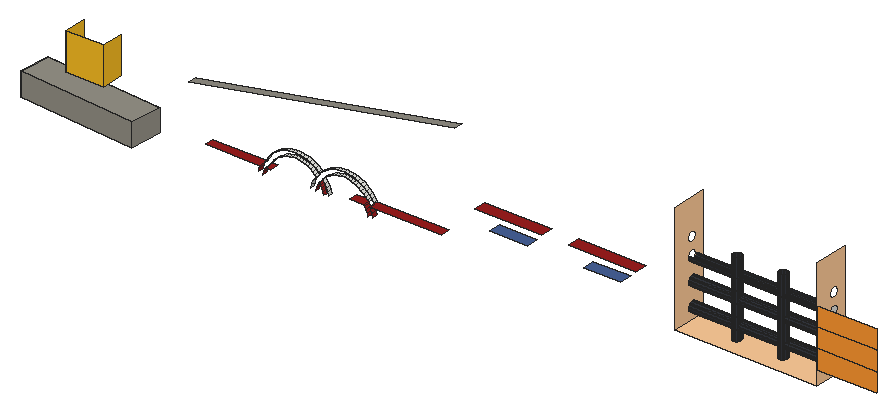
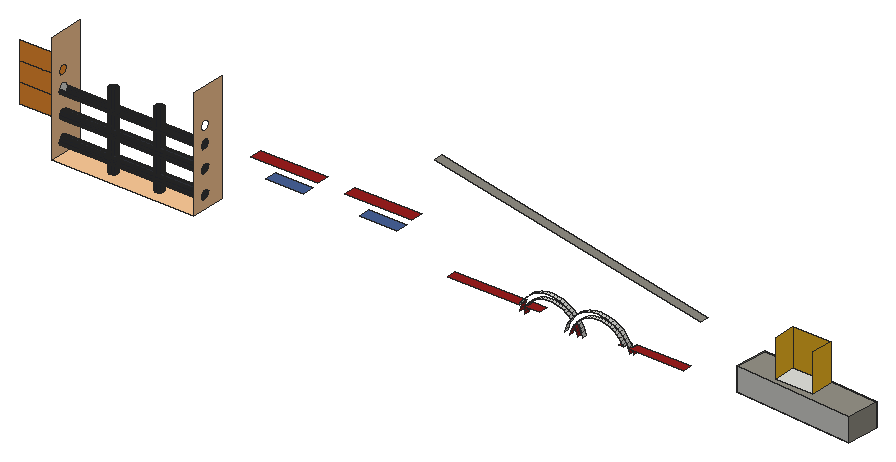
# SketchUp Ruby script. Lengths in inches.
U = 1.inch
M = Sketchup.active_model
def pt(a) = Geom::Point3d.new(a.map { |v| v * U })
def face(e, loops, mat)
  f = e.add_face(loops[0].map { |a| pt(a) })
  loops[1..].each { |l| e.add_face(l.map { |a| pt(a) }).erase! }
  f.material = f.back_material = mat if mat
  f
end
# faces: each face lists its corners as indices into pts; further lists are holes
def faces(e, pts, list, mat = nil) = list.each { |f| face(e, (f[0].is_a?(Array) ? f : [f]).map { |l| l.map { |i| pts[i] } }, mat) }
# xy, xz, yz: faces in a plane at the given z, y or x. An outline is a flat list of corners, or four numbers for a rectangle; further outlines are holes
def ring(l) = l.size == 4 ? [[l[0], l[1]], [l[2], l[1]], [l[2], l[3]], [l[0], l[3]]] : l.each_slice(2).to_a
def flat(e, list, mat, &to3) = list.each { |f| face(e, (f[0].is_a?(Array) ? f : [f]).map { |l| ring(l).map { |u, v| to3.(u, v) } }, mat) }
def xy(e, z, list, mat = nil) = flat(e, list, mat) { |x, y| [x, y, z] }
def xz(e, y, list, mat = nil) = flat(e, list, mat) { |x, z| [x, y, z] }
def yz(e, x, list, mat = nil) = flat(e, list, mat) { |y, z| [x, y, z] }
def lines(e, pts, list) = list.each { |a, b| e.add_line(pt(pts[a]), pt(pts[b])) }
# prism: a flat outline (further loops are holes) pulled along v
def prism(e, loops, v, mat = nil)
  f = face(e, loops, mat); d = Geom::Vector3d.new(v.map { |x| x * U })
  f.pushpull(f.normal.samedirection?(d) ? d.length : -d.length)
end
def box(e, o, s, mat = nil) = prism(e, [[o, [o[0] + s[0], o[1], o[2]], [o[0] + s[0], o[1] + s[1], o[2]], [o[0], o[1] + s[1], o[2]]]], [0, 0, s[2]], mat)
def at(x, y, z, deg = 0) = Geom::Transformation.translation(pt([x, y, z])) * Geom::Transformation.rotation(ORIGIN, Z_AXIS, deg.degrees)
def axes(o, x, y, z) = Geom::Transformation.new([*x, 0, *y, 0, *z, 0, *pt(o).to_a, 1])
def part(name) = M.definitions.add(name)
# library, detail: a bought-in or finely detailed component or shape, given as its bounding box
def library(name, o, s) = part(name).tap { |d| box(d.entities, o, s) }
def detail(e, o, s) = box(e.add_group.entities, o, s)
def put(e, d, t, mat = nil) = e.add_instance(d, t).tap { |i| i.material = mat if mat }
def group(e, t, mat = nil) = e.add_group.tap { |g| g.transformation = t; g.material = mat if mat }.entities
root = M.entities
M.materials.add("[0045_Goldenrod]").color = [249, 189, 36]
M.materials.add("[Color A04]").color = [155, 30, 30]
M.materials.add("[Color C02]").color = [255, 204, 153]
M.materials.add("[Color C04]").color = [255, 153, 50]
M.materials.add("[Formica Blue]").color = [71, 97, 152]
M.materials.add("[Formica Graystone]").color = [149, 146, 135]
M.materials.add("[Formica Laminate Dark]").color = [50, 53, 60]
xy(root,271.875,[[[383.64,94.74,470.23,116.19],[411.92,104.06,411.25,104.14,410.64,104.4,410.11,104.81,409.7,105.34,409.44,105.95,409.36,106.62,409.44,107.28,409.7,107.9,410.11,108.43,410.64,108.84,411.25,109.09,411.92,109.18,412.58,109.09,413.2,108.84,413.73,108.43,414.14,107.9,414.39,107.28,414.48,106.62,414.39,105.95,414.14,105.34,413.73,104.81,413.2,104.4,412.58,104.14],[440.11,104.06,439.44,104.14,438.82,104.4,438.29,104.81,437.89,105.34,437.63,105.95,437.54,106.62,437.63,107.28,437.89,107.9,438.29,108.43,438.82,108.84,439.44,109.09,440.11,109.18,440.77,109.09,441.39,108.84,441.92,108.43,442.32,107.9,442.58,107.28,442.67,106.62,442.58,105.95,442.32,105.34,441.92,104.81,441.39,104.4,440.77,104.14]]],"[Color C02]")
xy(root,272.99,[[72.23,70.04,0,75.36,1.43,94.74,73.65,89.43]])
xy(root,276.95,[[101.95,89.24,135.19,94.74],[138.52,89.24,141.51,94.74]],"[Color A04]")
xy(root,277.9375,[[189.67,89.24,198.57,94.74],[202,89.24,245.58,94.74]],"[Color A04]")
xy(root,287.03,[[72.23,70.04,73.65,89.43,1.43,94.74,0,75.36]],"[Formica Graystone]")
xy(root,291.97,[[276.8,87.3,299.68,94.74],[333.8,87.3,356.68,94.74]],"[Formica Blue]")
xy(root,292.05,[[23.1,81.43,45.78,94.74]])
xy(root,300.97,[[267.8,87.3,308.68,94.74],[324.8,87.3,365.68,94.74]],"[Color A04]")
xz(root,81.43,[[23.1,292.05,45.78,314.74]],"[0045_Goldenrod]")
xz(root,94.74,[[470.23,280.78,506.36,292.4],[470.23,292.4,506.36,304.03],[470.23,304.03,506.36,315.65]],"[Color C04]")
yz(root,23.1,[[81.43,292.05,94.74,314.74]],"[0045_Goldenrod]")
yz(root,45.78,[[81.43,292.05,94.74,314.74]],"[0045_Goldenrod]")
yz(root,383.64,[[[94.74,271.875,116.19,338.91],[107.5,314.66,106.75,314.76,106.06,315.05,105.46,315.51,105.01,316.1,104.72,316.79,104.62,317.54,104.72,318.28,105.01,318.98,105.46,319.57,106.06,320.03,106.75,320.32,107.5,320.41,108.24,320.32,108.93,320.03,109.53,319.57,109.99,318.98,110.27,318.28,110.37,317.54,110.27,316.79,109.99,316.1,109.53,315.51,108.93,315.05,108.24,314.76],[107.5,304.48,106.75,304.57,106.06,304.86,105.46,305.32,105.01,305.91,104.72,306.61,104.62,307.35,104.72,308.09,105.01,308.79,105.46,309.38,106.06,309.84,106.75,310.13,107.5,310.23,108.24,310.13,108.93,309.84,109.53,309.38,109.99,308.79,110.27,308.09,110.37,307.35,110.27,306.61,109.99,305.91,109.53,305.32,108.93,304.86,108.24,304.57],[107.5,290.91,106.75,291.01,106.06,291.3,105.46,291.76,105.01,292.35,104.72,293.04,104.62,293.79,104.72,294.53,105.01,295.23,105.46,295.82,106.06,296.28,106.75,296.57,107.5,296.66,108.24,296.57,108.93,296.28,109.53,295.82,109.99,295.23,110.27,294.53,110.37,293.79,110.27,293.04,109.99,292.35,109.53,291.76,108.93,291.3,108.24,291.01],[107.5,276.73,106.75,276.82,106.06,277.11,105.46,277.57,105.01,278.16,104.72,278.86,104.62,279.6,104.72,280.34,105.01,281.04,105.46,281.63,106.06,282.09,106.75,282.38,107.5,282.48,108.24,282.38,108.93,282.09,109.53,281.63,109.99,281.04,110.27,280.34,110.37,279.6,110.27,278.86,109.99,278.16,109.53,277.57,108.93,277.11,108.24,276.82]]],"[Color C02]")
yz(root,470.23,[[107.5,276.73,108.24,276.82,108.93,277.11,109.53,277.57,109.99,278.16,110.27,278.86,110.37,279.6,110.27,280.34,109.99,281.04,109.53,281.63,108.93,282.09,108.24,282.38,107.5,282.48,106.75,282.38,106.06,282.09,105.46,281.63,105.01,281.04,104.72,280.34,104.62,279.6,104.72,278.86,105.01,278.16,105.46,277.57,106.06,277.11,106.75,276.82],[107.5,290.91,108.24,291.01,108.93,291.3,109.53,291.76,109.99,292.35,110.27,293.04,110.37,293.79,110.27,294.53,109.99,295.23,109.53,295.82,108.93,296.28,108.24,296.57,107.5,296.66,106.75,296.57,106.06,296.28,105.46,295.82,105.01,295.23,104.72,294.53,104.62,293.79,104.72,293.04,105.01,292.35,105.46,291.76,106.06,291.3,106.75,291.01],[107.5,304.48,108.24,304.57,108.93,304.86,109.53,305.32,109.99,305.91,110.27,306.61,110.37,307.35,110.27,308.09,109.99,308.79,109.53,309.38,108.93,309.84,108.24,310.13,107.5,310.23,106.75,310.13,106.06,309.84,105.46,309.38,105.01,308.79,104.72,308.09,104.62,307.35,104.72,306.61,105.01,305.91,105.46,305.32,106.06,304.86,106.75,304.57]])
yz(root,470.23,[[[94.74,271.875,116.19,338.91],[107.5,276.73,108.24,276.82,108.93,277.11,109.53,277.57,109.99,278.16,110.27,278.86,110.37,279.6,110.27,280.34,109.99,281.04,109.53,281.63,108.93,282.09,108.24,282.38,107.5,282.48,106.75,282.38,106.06,282.09,105.46,281.63,105.01,281.04,104.72,280.34,104.62,279.6,104.72,278.86,105.01,278.16,105.46,277.57,106.06,277.11,106.75,276.82],[107.5,290.91,108.24,291.01,108.93,291.3,109.53,291.76,109.99,292.35,110.27,293.04,110.37,293.79,110.27,294.53,109.99,295.23,109.53,295.82,108.93,296.28,108.24,296.57,107.5,296.66,106.75,296.57,106.06,296.28,105.46,295.82,105.01,295.23,104.72,294.53,104.62,293.79,104.72,293.04,105.01,292.35,105.46,291.76,106.06,291.3,106.75,291.01],[107.5,304.48,108.24,304.57,108.93,304.86,109.53,305.32,109.99,305.91,110.27,306.61,110.37,307.35,110.27,308.09,109.99,308.79,109.53,309.38,108.93,309.84,108.24,310.13,107.5,310.23,106.75,310.13,106.06,309.84,105.46,309.38,105.01,308.79,104.72,308.09,104.62,307.35,104.72,306.61,105.01,305.91,105.46,305.32,106.06,304.86,106.75,304.57],[107.5,314.66,108.24,314.76,108.93,315.05,109.53,315.51,109.99,316.1,110.27,316.79,110.37,317.54,110.27,318.28,109.99,318.98,109.53,319.57,108.93,320.03,108.24,320.32,107.5,320.41,106.75,320.32,106.06,320.03,105.46,319.57,105.01,318.98,104.72,318.28,104.62,317.54,104.72,316.79,105.01,316.1,105.46,315.51,106.06,315.05,106.75,314.76]]],"[Color C02]")
p = [[410.64,104.4,271.875],[411.25,104.14,271.875],[411.25,104.14,317.54],[410.64,104.4,317.54],[411.92,104.06,271.875],[411.92,104.06,317.54],
  [412.58,104.14,271.875],[412.58,104.14,317.54],[413.2,104.4,271.875],[413.2,104.4,317.54],[438.82,104.4,271.875],[439.44,104.14,271.875],
  [439.44,104.14,318.0625],[438.82,104.4,318.0625],[440.11,104.06,271.875],[440.11,104.06,318.0625],[440.77,104.14,271.875],[440.77,104.14,318.0625],
  [441.39,104.4,271.875],[441.39,104.4,318.0625],[410.11,104.81,271.875],[410.35,104.62,317.54],[410.11,104.81,317.54],[413.73,104.81,271.875],
  [413.73,104.81,317.54],[413.49,104.62,317.54],[438.29,104.81,271.875],[438.29,104.81,318.0625],[441.92,104.81,271.875],[441.92,104.81,318.0625],
  [409.7,105.34,271.875],[409.7,105.34,317.54],[414.14,105.34,271.875],[414.14,105.34,317.54],[437.89,105.34,271.875],[437.89,105.34,318.0625],
  [442.32,105.34,271.875],[442.32,105.34,318.0625],[409.44,105.95,271.875],[409.44,105.95,317.54],[414.39,105.95,271.875],[414.39,105.95,317.54],
  [437.63,105.95,271.875],[437.63,105.95,318.0625],[442.58,105.95,271.875],[442.58,105.95,318.0625],[409.36,106.62,271.875],[409.36,106.62,317.54],
  [414.48,106.62,271.875],[414.48,106.62,317.54],[437.54,106.62,271.875],[437.54,106.62,318.0625],[442.67,106.62,271.875],[442.67,106.62,318.0625],
  [409.44,107.28,271.875],[409.44,107.28,317.54],[414.39,107.28,271.875],[414.39,107.28,317.54],[437.63,107.28,271.875],[437.63,107.28,318.0625],
  [442.58,107.28,271.875],[442.58,107.28,318.0625],[409.7,107.9,271.875],[409.7,107.9,317.54],[414.14,107.9,271.875],[414.14,107.9,317.54],
  [437.89,107.9,271.875],[437.89,107.9,318.0625],[442.32,107.9,271.875],[442.32,107.9,318.0625],[410.11,108.43,271.875],[410.11,108.43,317.54],
  [413.73,108.43,271.875],[413.73,108.43,317.54],[438.29,108.43,271.875],[438.29,108.43,318.0625],[441.92,108.43,271.875],[441.92,108.43,318.0625],
  [410.64,108.84,271.875],[410.64,108.84,317.54],[413.2,108.84,271.875],[413.2,108.84,317.54],[438.82,108.84,271.875],[438.82,108.84,318.0625],
  [441.39,108.84,271.875],[441.39,108.84,318.0625],[411.25,109.09,271.875],[411.25,109.09,317.54],[412.58,109.09,271.875],[412.58,109.09,317.54],
  [439.44,109.09,271.875],[439.44,109.09,318.0625],[440.77,109.09,271.875],[440.77,109.09,318.0625],[411.92,109.18,271.875],[411.92,109.18,317.54],
  [440.11,109.18,271.875],[440.11,109.18,318.0625],[200.89,92.37,272.03],[200.45,92.37,273.82],[200.45,89.24,273.82],[200.89,89.24,272.03],
  [170.95,94.74,273.82],[171.39,94.74,272.03],[171.39,92.37,272.03],[170.95,92.37,273.82],[203.32,92.37,274.6875],[203.84,92.37,272.59],
  [203.84,89.24,272.59],[203.32,89.24,274.6875],[174.34,94.74,272.59],[173.82,94.74,274.6875],[173.82,92.37,274.6875],[174.34,92.37,272.59],
  [136.92,92.37,272.73],[136.92,89.24,272.73],[137.43,89.24,274.51],[137.43,92.37,274.51],[166.42,94.74,272.73],[166.93,94.74,274.51],
  [166.93,92.37,274.51],[166.42,92.37,272.73],[72.23,70.04,287.03],[0,75.36,287.03],[0,75.36,272.99],[72.23,70.04,272.99],
  [73.65,89.43,272.99],[73.65,89.43,287.03],[1.43,94.74,287.03],[1.43,94.74,272.99],[134,92.37,273.42],[134.6,92.37,275.49],
  [134.6,89.24,275.49],[134,89.24,273.42],[164.1,94.74,275.49],[163.5,94.74,273.42],[163.5,92.37,273.42],[164.1,92.37,275.49],
  [199.82,92.37,275.55],[199.82,89.24,275.55],[170.32,94.74,275.55],[170.32,92.37,275.55],[138.13,89.24,276.21],[138.13,92.37,276.21],
  [167.63,94.74,276.21],[167.63,92.37,276.21],[202.59,92.37,276.72],[202.59,89.24,276.72],[173.09,94.74,276.72],[173.09,92.37,276.72],
  [135.19,92.37,276.95],[135.19,89.24,276.95],[164.91,94.74,277.49],[164.91,92.37,277.49],[199.02,92.37,277.21],[199.02,89.24,277.21],
  [169.52,94.74,277.21],[169.52,92.37,277.21],[138.52,89.24,276.95],[138.52,92.37,276.95],[168.5,94.74,277.84],[168.5,92.37,277.84],
  [202,92.37,277.9375],[202,89.24,277.9375],[172.15,94.74,278.66],[172.15,92.37,278.66],[470.23,107.5,276.73],[470.23,106.75,276.82],
  [383.64,106.75,276.82],[383.64,107.5,276.73],[470.23,108.24,276.82],[383.64,108.24,276.82],[470.23,106.06,277.11],[383.64,106.06,277.11],
  [470.23,108.93,277.11],[383.64,108.93,277.11],[135.41,94.74,277.49],[135.19,94.74,276.95],[135.41,92.37,277.49],[138.52,94.74,276.95],
  [139,94.74,277.84],[139,92.37,277.84],[470.23,105.46,277.57],[383.64,105.46,277.57],[470.23,109.53,277.57],[383.64,109.53,277.57],
  [198.57,92.37,277.9375],[198.57,89.24,277.9375],[168.83,94.74,278.32],[168.83,92.37,278.32],[136.43,94.74,279.39],[136.43,92.37,279.39],
  [165.93,94.74,279.39],[165.93,92.37,279.39],[470.23,105.01,278.16],[383.64,105.01,278.16],[470.23,109.99,278.16],[383.64,109.99,278.16],
  [140.04,94.74,279.37],[140.04,92.37,279.37],[198.04,94.74,278.78],[198.57,94.74,277.9375],[198.04,92.37,278.78],[202,94.74,277.9375],
  [201.65,94.74,278.66],[201.65,92.37,278.66],[470.23,104.72,278.86],[383.64,104.72,278.86],[470.23,110.27,278.86],[383.64,110.27,278.86],
  [171.01,94.74,280.5],[171.01,92.37,280.5],[200.51,94.74,280.5],[200.51,92.37,280.5],[196.91,94.74,280.24],[196.91,92.37,280.24],
  [470.23,104.62,279.6],[383.64,104.62,279.6],[470.23,110.37,279.6],[383.64,110.37,279.6],[137.64,94.74,281.18],[137.64,92.37,281.18],
  [141.23,94.74,280.78],[141.23,92.37,280.78],[166.88,94.74,280.79],[166.88,92.37,280.79],[470.23,104.72,280.34],[383.64,104.72,280.34],
  [470.23,110.27,280.34],[383.64,110.27,280.34],[195.64,94.74,281.57],[195.64,92.37,281.57],[470.23,105.01,281.04],[383.64,105.01,281.04],
  [470.23,109.99,281.04],[383.64,109.99,281.04],[170.76,94.74,280.8125],[170.76,92.37,280.8125],[199.19,94.74,282.2],[199.19,92.37,282.2],
  [142.56,94.74,282.05],[142.56,92.37,282.05],[166.14,94.74,281.57],[166.14,92.37,281.57],[172.06,94.74,282.05],[172.06,92.37,282.05],
  [470.23,105.46,281.63],[383.64,105.46,281.63],[470.23,109.53,281.63],[383.64,109.53,281.63],[139.04,94.74,282.83],[139.04,92.37,282.83],
  [164.73,94.74,282.76],[164.73,92.37,282.76],[194.23,94.74,282.76],[194.23,92.37,282.76],[470.23,106.06,282.09],[383.64,106.06,282.09],
  [470.23,108.93,282.09],[383.64,108.93,282.09],[144.01,94.74,283.18],[144.01,92.37,283.18],[173.51,94.74,283.18],[173.51,92.37,283.18],
  [470.23,106.75,282.38],[383.64,106.75,282.38],[470.23,108.24,282.38],[383.64,108.24,282.38],[197.69,94.74,283.76],[197.69,92.37,283.76],
  [470.23,107.5,282.48],[383.64,107.5,282.48],[140.59,94.74,284.32],[140.59,92.37,284.32],[163.2,94.74,283.8],[163.2,92.37,283.8],
  [192.7,94.74,283.8],[192.7,92.37,283.8],[168.82,94.74,283.1],[168.19,94.74,283.76],[168.19,92.37,283.76],[168.82,92.37,283.1],
  [170.09,94.74,284.32],[170.09,92.37,284.32],[145.58,94.74,284.16],[145.58,92.37,284.16],[175.08,94.74,284.16],[175.08,92.37,284.16],
  [161.57,94.74,284.67],[161.57,92.37,284.67],[166.54,94.74,285.15],[166.54,92.37,285.15],[191.07,94.74,284.67],[191.07,92.37,284.67],
  [196.04,94.74,285.15],[196.04,92.37,285.15],[147.24,94.74,284.96],[147.24,92.37,284.96],[176.74,94.74,284.96],[176.74,92.37,284.96],
  [142.3,94.74,285.65],[142.3,92.37,285.65],[171.8,94.74,285.65],[171.8,92.37,285.65],[159.87,94.74,285.36],[159.87,92.37,285.36],
  [189.37,94.74,285.36],[189.37,92.37,285.36],[148.98,94.74,285.59],[148.98,92.37,285.59],[178.48,94.74,285.59],[178.48,92.37,285.59],
  [164.75,94.74,286.36],[164.75,92.37,286.36],[194.25,94.74,286.36],[194.25,92.37,286.36],[158.09,94.74,285.88],[158.09,92.37,285.88],
  [187.59,94.74,285.88],[187.59,92.37,285.88],[144.13,94.74,286.79],[144.13,92.37,286.79],[150.77,94.74,286.03],[150.77,92.37,286.03],
  [173.63,94.74,286.79],[173.63,92.37,286.79],[180.27,94.74,286.03],[180.27,92.37,286.03],[156.28,94.74,286.2],[156.28,92.37,286.2],
  [185.78,94.74,286.2],[185.78,92.37,286.2],[152.6,94.74,286.28],[152.6,92.37,286.28],[182.1,94.74,286.28],[182.1,92.37,286.28],
  [154.4375,94.74,286.34],[154.4375,92.37,286.34],[183.9375,94.74,286.34],[183.9375,92.37,286.34],[162.85,94.74,287.38],[162.85,92.37,287.38],
  [192.35,94.74,287.38],[192.35,92.37,287.38],[146.08,94.74,287.73],[146.08,92.37,287.73],[175.58,94.74,287.73],[175.58,92.37,287.73],
  [160.85,94.74,288.2],[160.85,92.37,288.2],[190.35,94.74,288.2],[190.35,92.37,288.2],[148.11,94.74,288.46],[148.11,92.37,288.46],
  [177.61,94.74,288.46],[177.61,92.37,288.46],[158.78,94.74,288.8],[158.78,92.37,288.8],[188.28,94.74,288.8],[188.28,92.37,288.8],
  [150.2,94.74,288.98],[150.2,92.37,288.98],[179.7,94.74,288.98],[179.7,92.37,288.98],[156.65,94.74,289.18],[156.65,92.37,289.18],
  [186.15,94.74,289.18],[186.15,92.37,289.18],[152.34,94.74,289.27],[152.34,92.37,289.27],[181.84,94.74,289.27],[181.84,92.37,289.27],
  [154.5,94.74,289.34],[154.5,92.37,289.34],[184,94.74,289.34],[184,92.37,289.34],[470.23,107.5,290.91],[470.23,106.75,291.01],
  [383.64,106.75,291.01],[383.64,107.5,290.91],[470.23,108.24,291.01],[383.64,108.24,291.01],[470.23,106.06,291.3],[383.64,106.06,291.3],
  [470.23,108.93,291.3],[383.64,108.93,291.3],[470.23,105.46,291.76],[383.64,105.46,291.76],[470.23,109.53,291.76],[383.64,109.53,291.76],
  [470.23,105.01,292.35],[383.64,105.01,292.35],[470.23,109.99,292.35],[383.64,109.99,292.35],[470.23,104.72,293.04],[383.64,104.72,293.04],
  [470.23,110.27,293.04],[383.64,110.27,293.04],[470.23,104.62,293.79],[383.64,104.62,293.79],[470.23,110.37,293.79],[383.64,110.37,293.79],
  [470.23,104.72,294.53],[383.64,104.72,294.53],[470.23,110.27,294.53],[383.64,110.27,294.53],[470.23,105.01,295.23],[383.64,105.01,295.23],
  [470.23,109.99,295.23],[383.64,109.99,295.23],[470.23,105.46,295.82],[383.64,105.46,295.82],[470.23,109.53,295.82],[383.64,109.53,295.82],
  [470.23,106.06,296.28],[383.64,106.06,296.28],[470.23,108.93,296.28],[383.64,108.93,296.28],[470.23,106.75,296.57],[383.64,106.75,296.57],
  [470.23,108.24,296.57],[383.64,108.24,296.57],[470.23,107.5,296.66],[383.64,107.5,296.66],[470.23,107.5,304.48],[470.23,106.75,304.57],
  [383.64,106.75,304.57],[383.64,107.5,304.48],[470.23,108.24,304.57],[383.64,108.24,304.57],[470.23,106.06,304.86],[383.64,106.06,304.86],
  [470.23,108.93,304.86],[383.64,108.93,304.86],[470.23,105.46,305.32],[383.64,105.46,305.32],[470.23,109.53,305.32],[383.64,109.53,305.32],
  [470.23,105.01,305.91],[383.64,105.01,305.91],[470.23,109.99,305.91],[383.64,109.99,305.91],[470.23,104.72,306.61],[383.64,104.72,306.61],
  [470.23,110.27,306.61],[383.64,110.27,306.61],[470.23,104.62,307.35],[383.64,104.62,307.35],[470.23,110.37,307.35],[383.64,110.37,307.35],
  [91.53,94.74,307.22],[253.89,94.74,338.91],[253.89,89.43,338.91],[91.53,89.43,307.22],[470.23,104.72,308.09],[383.64,104.72,308.09],
  [470.23,110.27,308.09],[383.64,110.27,308.09]]
faces(root,p,[[0,1,2,3],[1,4,5,2],[4,6,7,5],[6,8,9,7],[10,11,12,13],[11,14,15,12],[14,16,17,15],[16,18,19,17],
  [20,0,3,21,22],[8,23,24,25,9],[26,10,13,27],[18,28,29,19],[30,20,22,31],[23,32,33,24],[34,26,27,35],[28,36,37,29],
  [38,30,31,39],[32,40,41,33],[42,34,35,43],[36,44,45,37],[46,38,39,47],[40,48,49,41],[50,42,43,51],[44,52,53,45],
  [54,46,47,55],[48,56,57,49],[58,50,51,59],[52,60,61,53],[62,54,55,63],[56,64,65,57],[66,58,59,67],[60,68,69,61],
  [70,62,63,71],[64,72,73,65],[74,66,67,75],[68,76,77,69],[78,70,71,79],[72,80,81,73],[82,74,75,83],[76,84,85,77],
  [86,78,79,87],[80,88,89,81],[90,82,83,91],[84,92,93,85],[94,86,87,95],[88,94,95,89],[96,90,91,97],[92,96,97,93],
  [166,167,168,169],[170,166,169,171],[167,172,173,168],[174,170,171,175],[172,182,183,173],[184,174,175,185],[182,194,195,183],[196,184,185,197],
  [194,206,207,195],[208,196,197,209],[206,216,217,207],[218,208,209,219],[216,226,227,217],[228,218,219,229],[226,232,233,227],[234,228,229,235],
  [232,246,247,233],[248,234,235,249],[246,256,257,247],[258,248,249,259],[256,264,265,257],[266,258,259,267],[264,270,271,265],[270,266,267,271],
  [376,377,378,379],[380,376,379,381],[377,382,383,378],[384,380,381,385],[382,386,387,383],[388,384,385,389],[386,390,391,387],[392,388,389,393],
  [390,394,395,391],[396,392,393,397],[394,398,399,395],[400,396,397,401],[398,402,403,399],[404,400,401,405],[402,406,407,403],[408,404,405,409],
  [406,410,411,407],[412,408,409,413],[410,414,415,411],[416,412,413,417],[414,418,419,415],[420,416,417,421],[418,422,423,419],[422,420,421,423],
  [424,425,426,427],[428,424,427,429],[425,430,431,426],[432,428,429,433],[430,434,435,431],[436,432,433,437],[434,438,439,435],[440,436,437,441],
  [438,442,443,439],[444,440,441,445],[442,446,447,443],[448,444,445,449],[446,454,455,447],[456,448,449,457]],"[Formica Laminate Dark]")
faces(root,p,[[98,99,100,101],[102,103,104,105],[106,107,108,109],[114,115,116,117],[118,119,120,121],[130,131,132,133],[99,138,139,100],[140,102,105,141],
  [117,116,142,143],[119,144,145,120],[146,106,109,147],[131,150,151,132],[138,154,155,139],[156,140,141,157],[143,142,158,159],[144,160,161,145],
  [162,146,147,163],[154,186,187,155],[188,156,157,189],[160,188,189,161]],"[Color A04]")
faces(root,p,[[110,111,112,113],[128,127,126,129],[134,135,136,137],[111,148,149,112],[152,134,137,153],[148,164,165,149],[176,177,150,178],[179,180,181,159],
  [190,176,178,191],[192,152,153,193],[180,198,199,181],[200,201,186,202],[203,204,205,162],[164,210,211,165],[204,212,213,205],[214,200,202,215],
  [220,190,191,221],[198,222,223,199],[224,192,193,225],[230,214,215,231],[210,236,237,211],[212,238,239,213],[222,240,241,223],[242,224,225,243],
  [236,244,245,237],[250,220,221,251],[252,242,243,253],[254,230,231,255],[240,260,261,241],[244,262,263,245],[238,268,269,239],[272,250,251,273],
  [274,252,253,275],[276,254,255,277],[278,279,280,281],[282,278,281,283],[260,284,285,261],[262,286,287,263],[288,274,275,289],[279,290,291,280],
  [292,276,277,293],[268,294,295,269],[284,296,297,285],[286,298,299,287],[300,272,273,301],[302,282,283,303],[304,288,289,305],[306,292,293,307],
  [296,308,309,297],[298,310,311,299],[290,312,313,291],[294,314,315,295],[316,304,305,317],[318,306,307,319],[320,300,301,321],[308,322,323,309],
  [324,302,303,325],[310,326,327,311],[328,316,317,329],[330,318,319,331],[322,332,333,323],[326,334,335,327],[336,328,329,337],[338,330,331,339],
  [332,336,337,333],[334,338,339,335],[312,340,341,313],[314,342,343,315],[344,320,321,345],[346,324,325,347],[340,348,349,341],[342,350,351,343],
  [352,344,345,353],[354,346,347,355],[348,356,357,349],[350,358,359,351],[360,352,353,361],[362,354,355,363],[356,364,365,357],[358,366,367,359],
  [368,360,361,369],[370,362,363,371],[364,372,373,365],[366,374,375,367],[372,368,369,373],[374,370,371,375]])
faces(root,p,[[122,123,124,125],[126,127,122,125],[128,129,124,123],[450,451,452,453]],"[Formica Graystone]")
